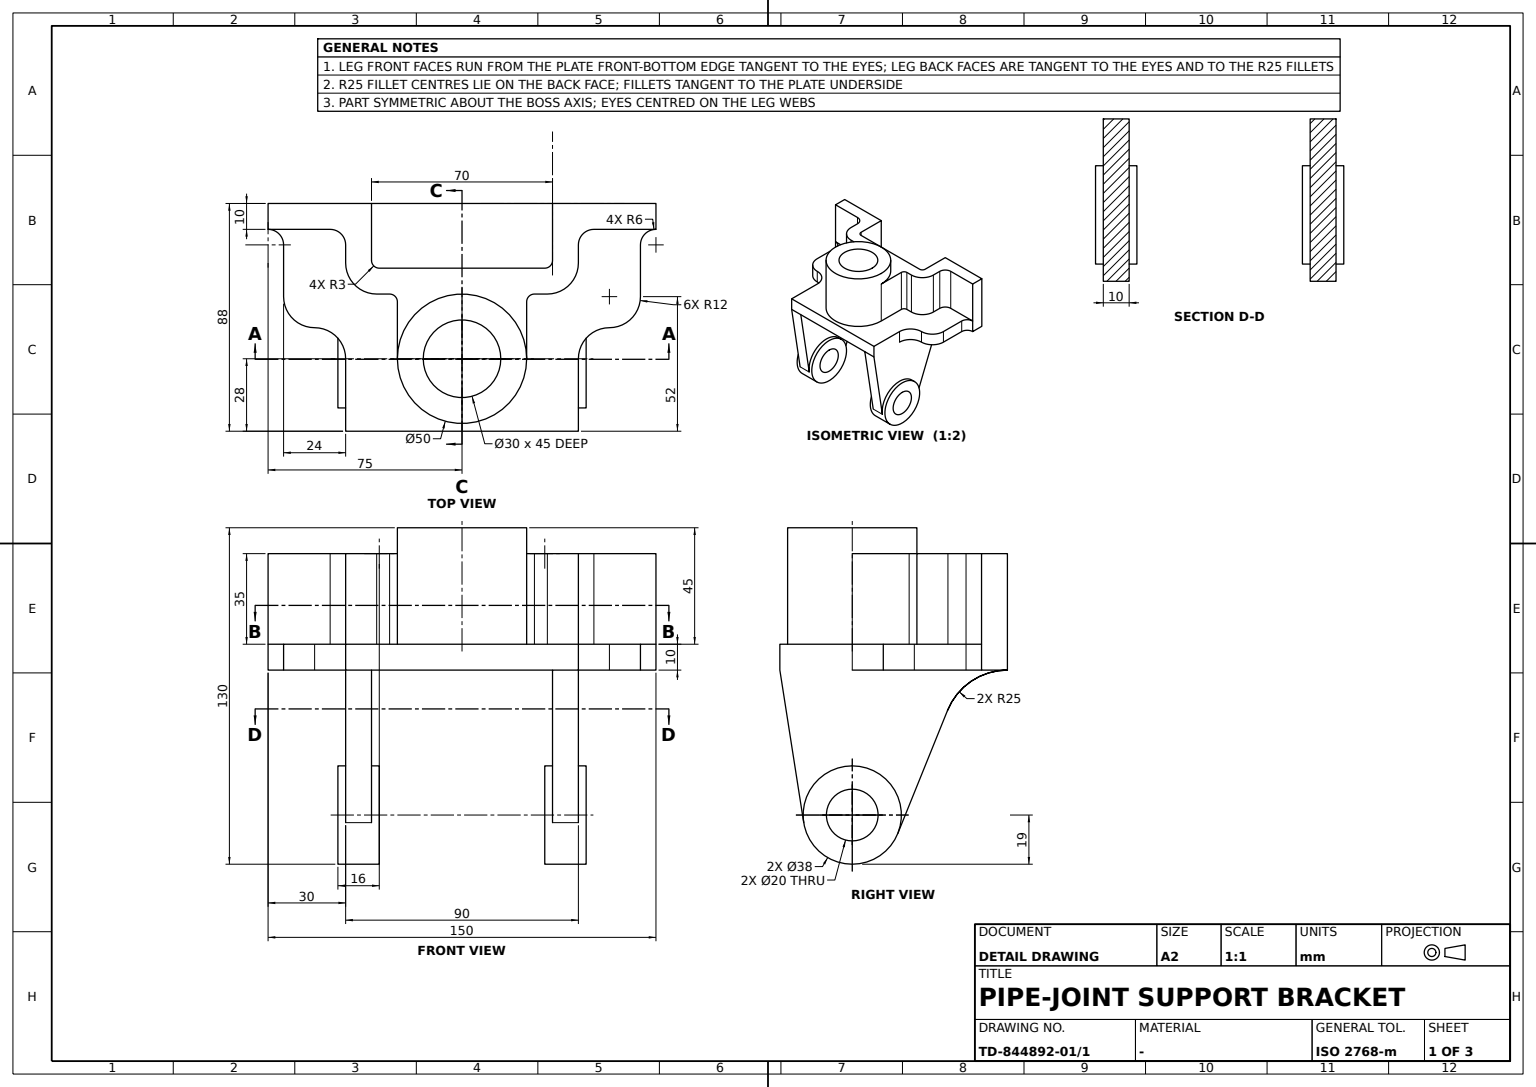
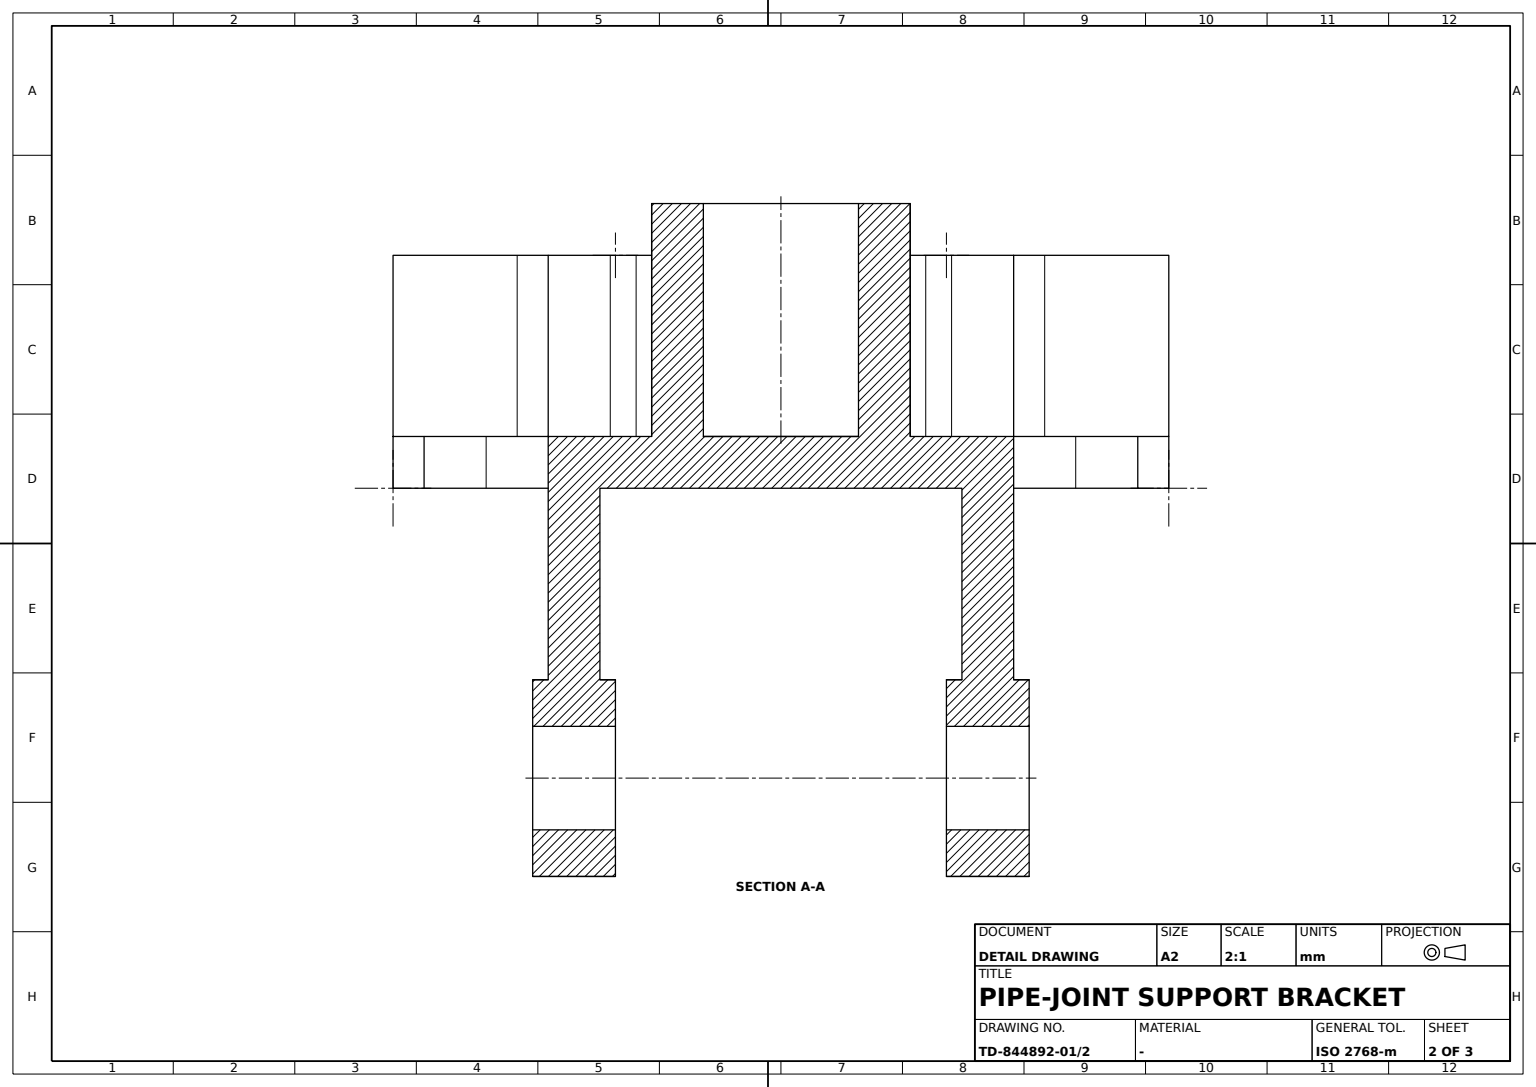
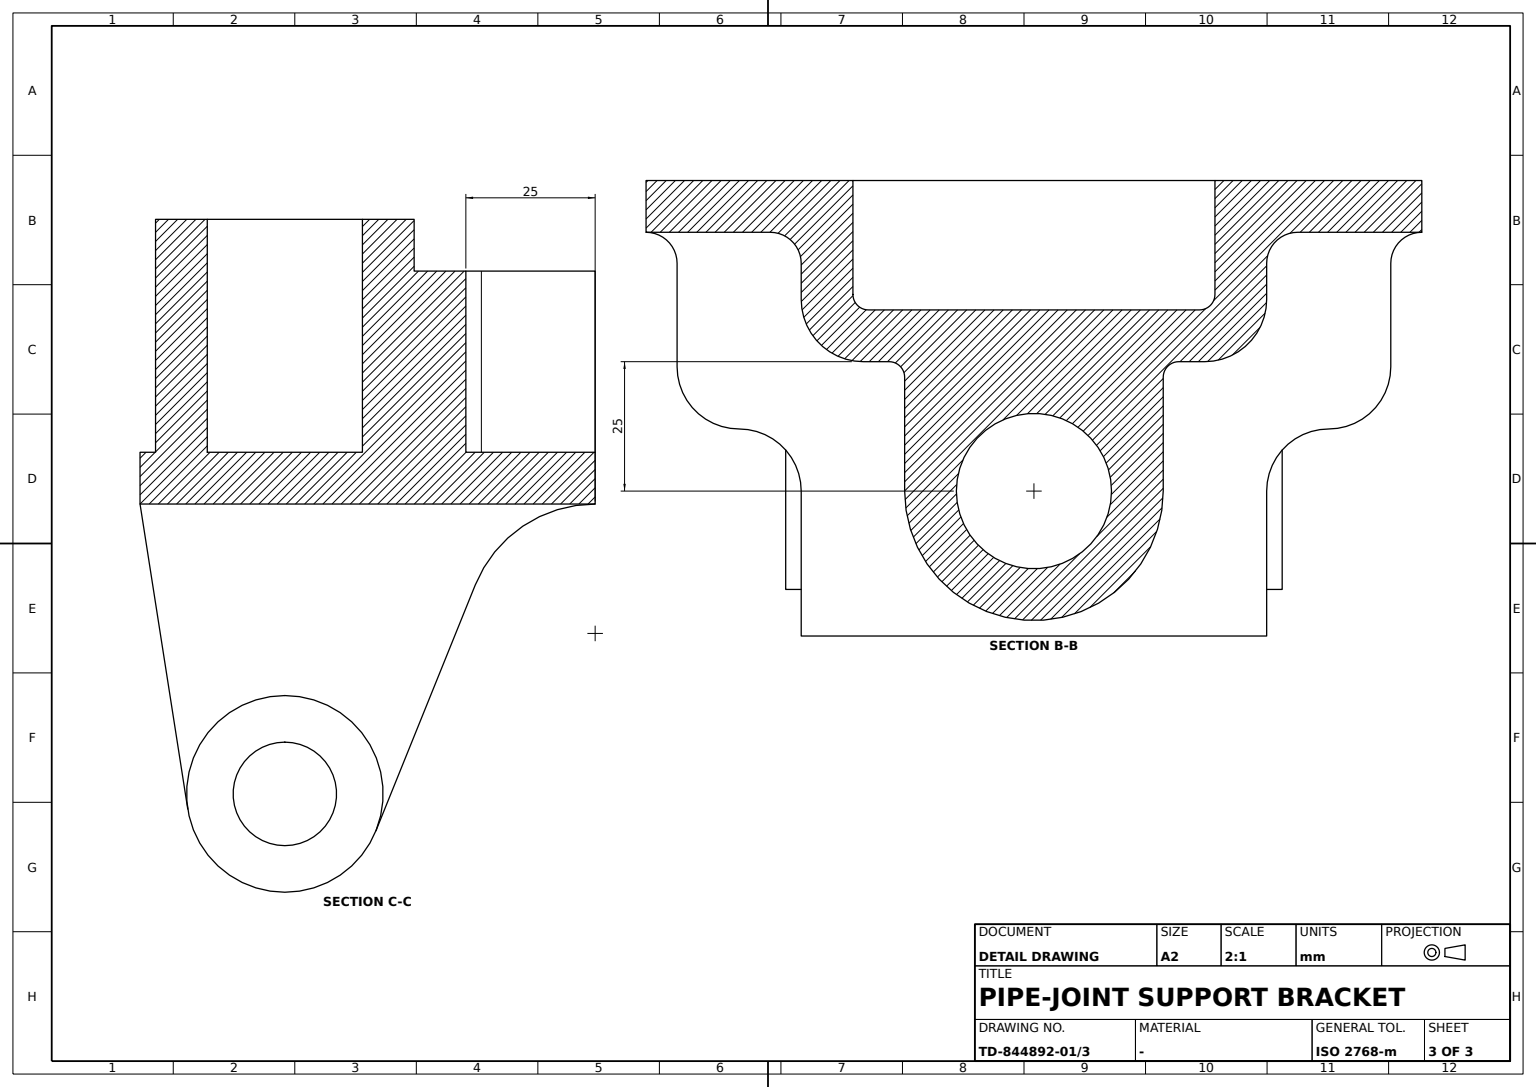
solid
v1 (33,53,10)
v2 (45,65,10)
e1 v1 v2 CIRCLE(AX(P(33,65,10),D(0,0,1),D(1,0,0)),12)
v3 (45,65,45)
e2 v2 v3 LINE
v4 (33,53,45)
e3 v4 v3 CIRCLE(AX(P(33,65,45),D(0,0,1),D(1,0,0)),12)
e4 v1 v4 LINE
face CYL(AX(P(33,65,27.5),D(0,0,1),D(1,0,0)),12) [e1 e2 -e3 -e4]
v5 (25,28,55)
e5 v5 v5 CIRCLE(AX(P(0,28,55),D(0,0,1),D(1,0,0)),25)
v6 (25,28,10)
v7 (25,28,45)
e6 v6 v7 LINE
v8 (-25,28,45)
e7 v7 v8 CIRCLE(AX(P(0,28,45),D(0,0,1),D(1,0,0)),25)
v9 (-25,28,10)
e8 v9 v8 LINE
e9 v9 v6 CIRCLE(AX(P(0,28,10),D(0,0,1),D(1,0,0)),25)
face CYL(AX(P(0,28,32.5),D(0,0,1),D(1,0,0)),25) [-e5] [e6 e7 -e8 e9]
v10 (51,78,45)
v11 (45,72,45)
e10 v10 v11 CIRCLE(AX(P(51,72,45),D(0,0,1),D(1,0,0)),6)
v12 (45,72,10)
e11 v12 v11 LINE
v13 (51,78,10)
e12 v13 v12 CIRCLE(AX(P(51,72,10),D(0,0,1),D(1,0,0)),6)
e13 v13 v10 LINE
face CYL(AX(P(51,72,27.5),D(0,0,1),D(1,0,0)),6) rev [e10 -e11 -e12 e13]
v14 (69,52,0)
v15 (69,52,10)
e14 v14 v15 LINE
v16 (69,72,0)
e15 v14 v16 LINE
v17 (69,72,10)
e16 v16 v17 LINE
e17 v15 v17 LINE
face PLANE(AX(P(69,40,0),D(1,0,0),D(0,1,0))) [-e14 e15 e16 -e17]
v18 (57,40,0)
e18 v18 v14 CIRCLE(AX(P(57,52,0),D(0,0,1),D(1,0,0)),12)
v19 (45,28,0)
e19 v18 v19 CIRCLE(AX(P(57,28,0),D(0,0,1),D(1,0,0)),12)
v20 (45,88,0)
e20 v19 v20 LINE
v21 (75,88,0)
e21 v20 v21 LINE
v22 (75,78,0)
e22 v22 v21 LINE
e23 v22 v16 CIRCLE(AX(P(75,72,0),D(0,0,1),D(1,0,0)),6)
face PLANE(AX(P(0,0,0),D(0,0,1),D(1,0,0))) rev [-e15 -e18 e19 e20 e21 -e22 e23]
v23 (-45,72,10)
v24 (-51,78,10)
e24 v23 v24 CIRCLE(AX(P(-51,72,10),D(0,0,1),D(1,0,0)),6)
v25 (-45,72,45)
e25 v23 v25 LINE
v26 (-51,78,45)
e26 v25 v26 CIRCLE(AX(P(-51,72,45),D(0,0,1),D(1,0,0)),6)
e27 v24 v26 LINE
face CYL(AX(P(-51,72,27.5),D(0,0,1),D(1,0,0)),6) rev [-e24 e25 e26 -e27]
v27 (35,9.228718,-58.939212)
v28 (45,9.228718,-58.939212)
e28 v27 v28 LINE
v29 (45,0,0)
e29 v29 v28 LINE
v30 (35,0,0)
e30 v29 v30 LINE
e31 v30 v27 LINE
face PLANE(AX(P(45,0,0),D(0,0.987962214,0.154695393),D(0,0.154695393,-0.987962214))) rev [e28 -e29 e30 e31]
v31 (-69,72,0)
v32 (-75,78,0)
e32 v31 v32 CIRCLE(AX(P(-75,72,0),D(0,0,1),D(1,0,0)),6)
v33 (-75,88,0)
e33 v32 v33 LINE
v34 (-45,88,0)
e34 v33 v34 LINE
v35 (-45,28,0)
e35 v35 v34 LINE
v36 (-57,40,0)
e36 v35 v36 CIRCLE(AX(P(-57,28,0),D(0,0,1),D(1,0,0)),12)
v37 (-69,52,0)
e37 v37 v36 CIRCLE(AX(P(-57,52,0),D(0,0,1),D(1,0,0)),12)
e38 v37 v31 LINE
face PLANE(AX(P(0,0,0),D(0,0,1),D(1,0,0))) rev [e32 e33 e34 -e35 e36 -e37 e38]
v38 (48,28,-37)
e39 v38 v38 CIRCLE(AX(P(48,28,-56),D(-1,0,0),D(0,0,1)),19)
v39 (48,28,-46)
e40 v39 v39 CIRCLE(AX(P(48,28,-56),D(-1,0,0),D(0,0,1)),10)
face PLANE(AX(P(48,0,0),D(-1,0,0),D(0,-1,0))) rev [-e39] [e40]
v40 (-35,0,0)
v41 (-35,88,0)
e41 v40 v41 LINE
v42 (35,88,0)
e42 v41 v42 LINE
e43 v30 v42 LINE
e44 v40 v30 LINE
face PLANE(AX(P(0,0,0),D(0,0,1),D(1,0,0))) rev [e41 e42 -e43 -e44]
v43 (-48,28,-37)
e45 v43 v43 CIRCLE(AX(P(-48,28,-56),D(-1,0,0),D(0,0,1)),19)
v44 (-45,45.61396,-63.123793)
v45 (-45,9.228718,-58.939212)
e46 v44 v45 CIRCLE(AX(P(-45,28,-56),D(1,0,0),D(0,0,-1)),19)
v46 (-35,45.61396,-63.123793)
e47 v44 v46 LINE
v47 (-35,9.228718,-58.939212)
e48 v46 v47 CIRCLE(AX(P(-35,28,-56),D(-1,0,0),D(0,0,1)),19) rev
e49 v45 v47 LINE
v48 (-32,28,-37)
e50 v48 v48 CIRCLE(AX(P(-32,28,-56),D(-1,0,0),D(0,0,1)),19)
face CYL(AX(P(40,28,-56),D(-1,0,0),D(0,-1,0)),19) [-e45] [-e46 e47 e48 -e49] [e50]
v49 (57,40,10)
e51 v49 v15 CIRCLE(AX(P(57,52,10),D(0,0,1),D(1,0,0)),12)
e52 v18 v49 LINE
face CYL(AX(P(57,52,5),D(0,0,1),D(1,0,0)),12) [e18 e14 -e51 -e52]
v50 (-75,78,10)
e53 v32 v50 LINE
v51 (-75,78,45)
e54 v50 v51 LINE
v52 (-75,88,45)
e55 v52 v51 LINE
e56 v33 v52 LINE
face PLANE(AX(P(-75,78,0),D(1,0,0),D(0,1,0))) rev [e53 e54 -e55 -e56 -e33]
v53 (45,64.823737,-15.626588)
v54 (35,64.823737,-15.626588)
e57 v53 v54 LINE
v55 (45,45.61396,-63.123793)
e58 v55 v53 LINE
v56 (35,45.61396,-63.123793)
e59 v56 v55 LINE
e60 v56 v54 LINE
face PLANE(AX(P(45,45.61396,-63.123793),D(0,-0.927050508,0.374936468),D(0,0.374936468,0.927050508))) rev [-e57 -e58 -e59 e60]
v57 (-45,28,10)
v58 (-57,40,10)
e61 v57 v58 CIRCLE(AX(P(-57,28,10),D(0,0,1),D(1,0,0)),12)
e62 v36 v58 LINE
e63 v35 v57 LINE
face CYL(AX(P(-57,28,5),D(0,0,1),D(1,0,0)),12) rev [e61 -e62 -e36 e63]
v59 (15,28,10)
e64 v59 v59 CIRCLE(AX(P(0,28,10),D(0,0,1),D(1,0,0)),15)
face PLANE(AX(P(0,0,10),D(0,0,1),D(1,0,0))) [e64]
v60 (-45,0,0)
e65 v60 v45 LINE
e66 v40 v47 LINE
e67 v60 v40 LINE
face PLANE(AX(P(45,0,0),D(0,0.987962214,0.154695393),D(0,0.154695393,-0.987962214))) rev [e65 e49 -e66 -e67]
v61 (15,28,55)
e68 v61 v61 CIRCLE(AX(P(0,28,55),D(0,0,1),D(1,0,0)),15)
face CYL(AX(P(0,28,32.5),D(0,0,1),D(1,0,0)),15) rev [e68] [-e64]
v62 (45,0,10)
e69 v29 v62 LINE
e70 v55 v28 CIRCLE(AX(P(45,28,-56),D(1,0,0),D(0,0,-1)),19)
e71 v20 v53 CIRCLE(AX(P(45,88,-25),D(1,0,0),D(0,0,-1)),25)
v63 (45,28,10)
e72 v19 v63 LINE
e73 v62 v63 LINE
face PLANE(AX(P(45,0,0),D(1,0,0),D(0,1,0))) [-e69 e29 -e70 e58 -e71 -e20 e72 -e73]
v64 (-48,28,-46)
e74 v64 v64 CIRCLE(AX(P(-48,28,-56),D(-1,0,0),D(0,0,1)),10)
v65 (-32,28,-46)
e75 v65 v65 CIRCLE(AX(P(-32,28,-56),D(-1,0,0),D(0,0,1)),10)
face CYL(AX(P(40,28,-56),D(-1,0,0),D(0,-1,0)),10) rev [e74] [-e75]
v66 (32,28,-46)
e76 v66 v66 CIRCLE(AX(P(32,28,-56),D(-1,0,0),D(0,0,1)),10)
face CYL(AX(P(40,28,-56),D(-1,0,0),D(0,-1,0)),10) rev [e76] [-e40]
v67 (75,78,10)
e77 v67 v13 LINE
v68 (75,78,45)
e78 v67 v68 LINE
e79 v68 v10 LINE
face PLANE(AX(P(-75,78,10),D(0,-1,0),D(1,0,0))) [-e13 -e77 e78 e79]
v69 (-35,64.823737,-15.626588)
e80 v41 v69 CIRCLE(AX(P(-35,88,-25),D(-1,0,0),D(0,0,1)),25) rev
e81 v46 v69 LINE
face PLANE(AX(P(-35,88,10),D(-1,0,0),D(0,-1,0))) rev [-e80 -e41 e66 -e48 e81]
v70 (-45,64.823737,-15.626588)
e82 v44 v70 LINE
e83 v70 v69 LINE
face PLANE(AX(P(45,45.61396,-63.123793),D(0,-0.927050508,0.374936468),D(0,0.374936468,0.927050508))) rev [-e81 -e47 e82 e83]
e84 v22 v67 LINE
v71 (75,88,45)
e85 v21 v71 LINE
e86 v71 v68 LINE
face PLANE(AX(P(75,78,0),D(1,0,0),D(0,1,0))) [-e78 -e84 e22 e85 e86]
e87 v42 v54 CIRCLE(AX(P(35,88,-25),D(-1,0,0),D(0,0,1)),25) rev
e88 v56 v27 CIRCLE(AX(P(35,28,-56),D(-1,0,0),D(0,0,1)),19) rev
face PLANE(AX(P(35,88,10),D(-1,0,0),D(0,-1,0))) [-e31 e43 e87 -e60 e88]
v72 (-45,0,10)
e89 v72 v57 LINE
e90 v34 v70 CIRCLE(AX(P(-45,88,-25),D(1,0,0),D(0,0,-1)),25)
e91 v60 v72 LINE
face PLANE(AX(P(-45,0,0),D(1,0,0),D(0,1,0))) rev [e89 -e63 e35 e90 -e82 e46 -e65 e91]
v73 (28,53,10)
v74 (28,53,45)
e92 v73 v74 LINE
e93 v1 v73 LINE
e94 v4 v74 LINE
face PLANE(AX(P(-33,53,10),D(0,-1,0),D(1,0,0))) [-e92 -e93 e4 e94]
v75 (-35,66,10)
v76 (-35,66,45)
e95 v75 v76 LINE
v77 (-32,63,45)
e96 v76 v77 CIRCLE(AX(P(-32,66,45),D(0,0,1),D(1,0,0)),3)
v78 (-32,63,10)
e97 v78 v77 LINE
e98 v75 v78 CIRCLE(AX(P(-32,66,10),D(0,0,1),D(1,0,0)),3)
face CYL(AX(P(-32,66,27.5),D(0,0,1),D(1,0,0)),3) rev [e95 e96 -e97 -e98]
e99 v11 v3 LINE
v79 (35,88,45)
e100 v79 v71 LINE
v80 (35,66,45)
e101 v79 v80 LINE
v81 (32,63,45)
e102 v81 v80 CIRCLE(AX(P(32,66,45),D(0,0,1),D(1,0,0)),3)
e103 v77 v81 LINE
v82 (-35,88,45)
e104 v82 v76 LINE
e105 v52 v82 LINE
e106 v51 v26 LINE
v83 (-45,65,45)
e107 v25 v83 LINE
v84 (-33,53,45)
e108 v83 v84 CIRCLE(AX(P(-33,65,45),D(0,0,1),D(1,0,0)),12)
v85 (-28,53,45)
e109 v84 v85 LINE
v86 (-25,50,45)
e110 v86 v85 CIRCLE(AX(P(-28,50,45),D(0,0,1),D(1,0,0)),3)
e111 v8 v86 LINE
v87 (25,50,45)
e112 v7 v87 LINE
e113 v74 v87 CIRCLE(AX(P(28,50,45),D(0,0,1),D(1,0,0)),3)
face PLANE(AX(P(0,0,45),D(0,0,1),D(1,0,0))) [-e99 -e10 -e79 -e86 -e100 e101 -e102 -e103 -e96 -e104 -e105 e55 e106 -e26 e107 e108 e109 -e110 -e111 -e7 e112 -e113 -e94 e3]
v88 (25,50,10)
e114 v6 v88 LINE
e115 v88 v87 LINE
face PLANE(AX(P(25,28,10),D(1,0,0),D(0,1,0))) [-e6 e114 e115 -e112]
v89 (-25,50,10)
e116 v89 v86 LINE
e117 v9 v89 LINE
face PLANE(AX(P(-25,28,10),D(1,0,0),D(0,1,0))) rev [e8 e111 -e116 -e117]
e118 v73 v88 CIRCLE(AX(P(28,50,10),D(0,0,1),D(1,0,0)),3)
face CYL(AX(P(28,50,27.5),D(0,0,1),D(1,0,0)),3) rev [e113 -e115 -e118 e92]
face PLANE(AX(P(-32,0,0),D(-1,0,0),D(0,-1,0))) rev [-e50] [e75]
e119 v72 v62 LINE
face PLANE(AX(P(-45,0,0),D(0,-1,0),D(1,0,0))) [e44 -e30 e69 -e119 -e91 e67]
v90 (-45,65,10)
e120 v23 v90 LINE
e121 v90 v83 LINE
face PLANE(AX(P(-45,0,0),D(1,0,0),D(0,1,0))) rev [e120 e121 -e107 -e25]
v91 (-33,53,10)
e122 v90 v91 CIRCLE(AX(P(-33,65,10),D(0,0,1),D(1,0,0)),12)
e123 v91 v84 LINE
face CYL(AX(P(-33,65,27.5),D(0,0,1),D(1,0,0)),12) [e122 e123 -e108 -e121]
v92 (-69,52,10)
e124 v92 v58 CIRCLE(AX(P(-57,52,10),D(0,0,1),D(1,0,0)),12)
e125 v37 v92 LINE
face CYL(AX(P(-57,52,5),D(0,0,1),D(0,-1,0)),12) [e37 e62 -e124 -e125]
e126 v67 v17 CIRCLE(AX(P(75,72,10),D(0,0,1),D(1,0,0)),6)
face CYL(AX(P(75,72,5),D(0,0,1),D(0,1,0)),6) rev [e126 -e16 -e23 e84]
v93 (35,66,10)
e127 v93 v80 LINE
v94 (35,88,10)
e128 v94 v79 LINE
e129 v94 v93 LINE
face PLANE(AX(P(35,88,10),D(-1,0,0),D(0,-1,0))) [e127 -e101 -e128 e129]
e130 v12 v2 LINE
v95 (-28,53,10)
e131 v89 v95 CIRCLE(AX(P(-28,50,10),D(0,0,1),D(1,0,0)),3)
e132 v91 v95 LINE
e133 v50 v24 LINE
v96 (-69,72,10)
e134 v96 v50 CIRCLE(AX(P(-75,72,10),D(0,0,1),D(1,0,0)),6)
e135 v92 v96 LINE
e136 v49 v63 CIRCLE(AX(P(57,28,10),D(0,0,1),D(1,0,0)),12)
face PLANE(AX(P(0,0,10),D(0,0,1),D(1,0,0))) [-e126 e77 e12 e130 -e1 e93 e118 -e114 -e9 e117 e131 -e132 -e122 -e120 e24 -e133 -e134 -e135 e124 -e61 -e89 e119 e73 -e136 e51 e17]
v97 (32,28,-37)
e137 v97 v97 CIRCLE(AX(P(32,28,-56),D(-1,0,0),D(0,0,1)),19)
face CYL(AX(P(40,28,-56),D(-1,0,0),D(0,-1,0)),19) [-e137] [e39] [e70 -e28 -e88 e59]
e138 v31 v96 LINE
face CYL(AX(P(-75,72,5),D(0,0,1),D(1,0,0)),6) rev [-e32 e138 e134 -e53]
v98 (-35,88,10)
e139 v98 v75 LINE
e140 v98 v82 LINE
face PLANE(AX(P(-35,88,10),D(-1,0,0),D(0,-1,0))) rev [-e139 e140 e104 -e95]
e141 v20 v42 LINE
face CYL(AX(P(40,88,-25),D(1,0,0),D(0,1,0)),25) rev [e57 -e87 -e141 e71]
e142 v34 v41 LINE
face CYL(AX(P(40,88,-25),D(1,0,0),D(0,1,0)),25) rev [e80 -e83 -e90 e142]
face PLANE(AX(P(-75,78,10),D(0,-1,0),D(1,0,0))) [-e106 -e54 e133 e27]
face PLANE(AX(P(-48,0,0),D(-1,0,0),D(0,-1,0))) [-e74] [e45]
v99 (32,63,10)
e143 v99 v93 CIRCLE(AX(P(32,66,10),D(0,0,1),D(1,0,0)),3)
e144 v99 v81 LINE
face CYL(AX(P(32,66,27.5),D(0,0,1),D(1,0,0)),3) rev [-e127 -e143 e144 e102]
e145 v95 v85 LINE
face PLANE(AX(P(-33,53,10),D(0,-1,0),D(1,0,0))) [-e109 -e123 e132 e145]
face PLANE(AX(P(45,0,0),D(1,0,0),D(0,1,0))) [-e2 -e130 e11 e99]
e146 v98 v94 LINE
e147 v78 v99 LINE
face PLANE(AX(P(0,0,10),D(0,0,1),D(1,0,0))) [e143 -e129 -e146 e139 e98 e147]
face PLANE(AX(P(0,0,55),D(0,0,1),D(1,0,0))) [-e68] [e5]
face PLANE(AX(P(-32,63,10),D(0,-1,0),D(1,0,0))) rev [e103 -e144 -e147 e97]
face PLANE(AX(P(-69,40,0),D(1,0,0),D(0,1,0))) rev [e135 -e138 -e38 e125]
face CYL(AX(P(57,28,5),D(0,0,1),D(0,1,0)),12) rev [e52 e136 -e72 -e19]
face CYL(AX(P(-28,50,27.5),D(0,0,1),D(1,0,0)),3) rev [-e145 -e131 e116 e110]
face PLANE(AX(P(32,0,0),D(-1,0,0),D(0,-1,0))) [-e76] [e137]
face PLANE(AX(P(-75,88,0),D(0,-1,0),D(1,0,0))) rev [-e42 -e142 -e34 e56 e105 -e140 e146 e128 e100 -e85 -e21 e141]
